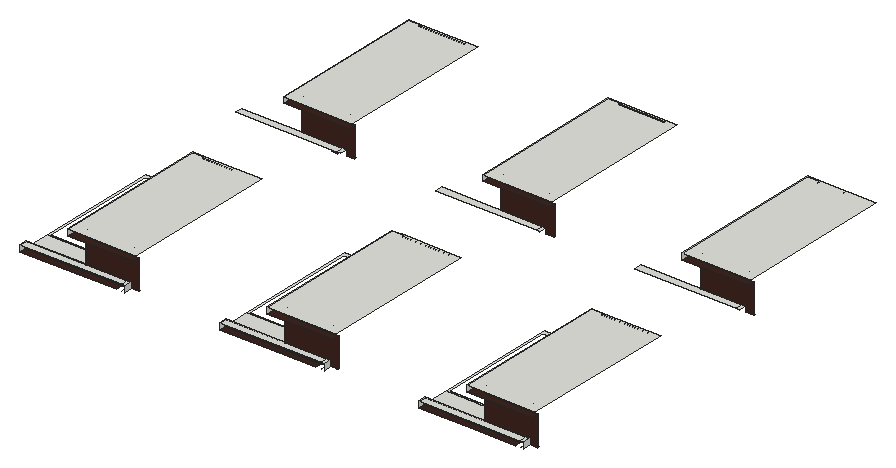
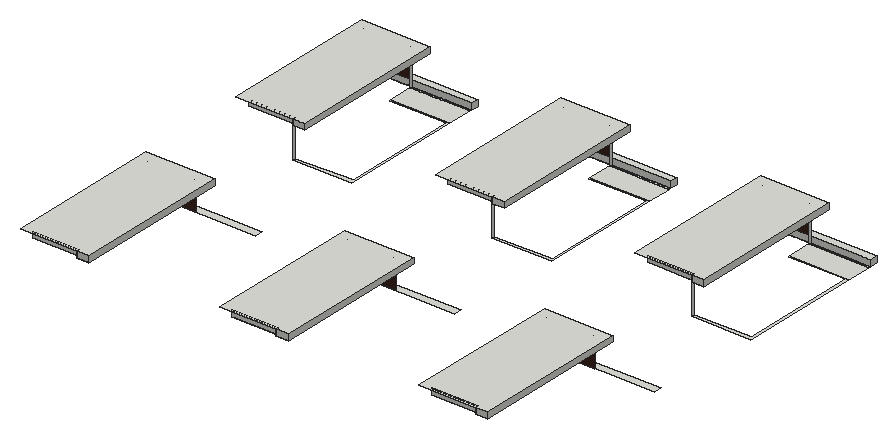
# SketchUp Ruby script. Lengths in inches.
U = 1.inch
M = Sketchup.active_model
def pt(a) = Geom::Point3d.new(a.map { |v| v * U })
def face(e, loops, mat)
  f = e.add_face(loops[0].map { |a| pt(a) })
  loops[1..].each { |l| e.add_face(l.map { |a| pt(a) }).erase! }
  f.material = f.back_material = mat if mat
  f
end
# faces: each face lists its corners as indices into pts; further lists are holes
def faces(e, pts, list, mat = nil) = list.each { |f| face(e, (f[0].is_a?(Array) ? f : [f]).map { |l| l.map { |i| pts[i] } }, mat) }
# xy, xz, yz: faces in a plane at the given z, y or x. An outline is a flat list of corners, or four numbers for a rectangle; further outlines are holes
def ring(l) = l.size == 4 ? [[l[0], l[1]], [l[2], l[1]], [l[2], l[3]], [l[0], l[3]]] : l.each_slice(2).to_a
def flat(e, list, mat, &to3) = list.each { |f| face(e, (f[0].is_a?(Array) ? f : [f]).map { |l| ring(l).map { |u, v| to3.(u, v) } }, mat) }
def xy(e, z, list, mat = nil) = flat(e, list, mat) { |x, y| [x, y, z] }
def xz(e, y, list, mat = nil) = flat(e, list, mat) { |x, z| [x, y, z] }
def yz(e, x, list, mat = nil) = flat(e, list, mat) { |y, z| [x, y, z] }
def lines(e, pts, list) = list.each { |a, b| e.add_line(pt(pts[a]), pt(pts[b])) }
# prism: a flat outline (further loops are holes) pulled along v
def prism(e, loops, v, mat = nil)
  f = face(e, loops, mat); d = Geom::Vector3d.new(v.map { |x| x * U })
  f.pushpull(f.normal.samedirection?(d) ? d.length : -d.length)
end
def box(e, o, s, mat = nil) = prism(e, [[o, [o[0] + s[0], o[1], o[2]], [o[0] + s[0], o[1] + s[1], o[2]], [o[0], o[1] + s[1], o[2]]]], [0, 0, s[2]], mat)
def at(x, y, z, deg = 0) = Geom::Transformation.translation(pt([x, y, z])) * Geom::Transformation.rotation(ORIGIN, Z_AXIS, deg.degrees)
def axes(o, x, y, z) = Geom::Transformation.new([*x, 0, *y, 0, *z, 0, *pt(o).to_a, 1])
def part(name) = M.definitions.add(name)
# library, detail: a bought-in or finely detailed component or shape, given as its bounding box
def library(name, o, s) = part(name).tap { |d| box(d.entities, o, s) }
def detail(e, o, s) = box(e.add_group.entities, o, s)
def put(e, d, t, mat = nil) = e.add_instance(d, t).tap { |i| i.material = mat if mat }
def group(e, t, mat = nil) = e.add_group.tap { |g| g.transformation = t; g.material = mat if mat }.entities
root = M.entities
M.materials.add("[0043_SaddleBrown]").color = [63, 38, 31]
xy(root,733.125,[[137.6,437.1,139.16,438.72],[139.16,437.1,143.93,438.72],[147.91,437.1,149.47,438.72],[149.47,437.1,154.24,438.72],[156.8,437.1,158.36,438.72],
  [158.36,437.1,163.14,438.72],[165.69,437.1,167.25,438.72],[167.25,437.1,172.03,438.72],[174.59,437.1,176.14,438.72],[176.14,437.1,180.92,438.72],
  [183.48,437.1,185.03,438.72],[185.03,437.1,189.81,438.72],[192.37,437.1,193.92,438.72],[193.92,437.1,198.7,438.72],[201.26,437.1,202.82,438.72],
  [202.82,437.1,207.59,438.72],[210.15,437.1,211.71,438.72],[211.71,437.1,216.48,438.72],[219.04,437.1,220.6,438.72],[220.6,437.1,225.375,438.72],
  [227.93,437.1,229.49,438.72],[229.49,437.1,234.27,438.72],[236.82,437.1,238.38,438.72],[238.38,437.1,243.16,438.72],[245.72,437.1,247.27,438.72],
  [247.27,437.1,252.05,438.72],[254.61,437.1,256.16,438.72],[256.16,437.1,260.94,438.72],[263.5,437.1,265.05,438.72],[265.05,437.1,269.83,438.72],
  [272.39,437.1,273.95,438.72],[273.95,437.1,278.72,438.72],[281.28,437.1,282.84,438.72],[282.84,437.1,287.61,438.72],[290.17,437.1,291.73,438.72],
  [291.73,437.1,296.51,438.72],[299.0625,437.1,300.62,438.72],[300.62,437.1,305.4,438.72],[307.95,437.1,309.51,438.72],[309.51,437.1,314.29,438.72],
  [316.85,437.1,318.4,438.72],[318.4,437.1,323.18,438.72],[325.74,437.1,327.29,438.72],[327.29,437.1,332.07,438.72],[334.63,437.1,336.19,438.72],
  [336.19,437.1,340.96,438.72],[343.52,437.1,345.08,438.72],[345.08,437.1,349.85,438.72],[352.41,437.1,353.97,438.72],[353.97,437.1,358.74,438.72],
  [361.3,437.1,367.0625,438.72],[369.3,437.1,375.0625,438.72],[377.3,437.1,383.0625,438.72],[385.3,437.1,391.0625,438.72],[393.3,437.1,399.0625,438.72],
  [401.3,437.1,407.0625,438.72],[409.3,437.1,415.0625,438.72],[417.3,437.1,423.0625,438.72],[425.3,437.1,431.0625,438.72],[433.3,437.1,439.0625,438.72],
  [441.3,437.1,447.0625,438.72],[449.3,437.1,455.0625,438.72],[457.3,437.1,463.0625,438.72],[465.3,437.1,471.0625,438.72],[473.3,437.1,479.0625,438.72],
  [481.3,437.1,487.0625,438.72],[862.04,437.1,863.59,438.72],[863.59,437.1,868.37,438.72],[872.35,437.1,873.91,438.72],[873.91,437.1,878.68,438.72],
  [881.24,437.1,882.8,438.72],[882.8,437.1,887.57,438.72],[890.13,437.1,891.6875,438.72],[891.6875,437.1,896.47,438.72],[899.02,437.1,900.58,438.72],
  [900.58,437.1,905.36,438.72],[907.91,437.1,909.47,438.72],[909.47,437.1,914.25,438.72],[916.81,437.1,918.36,438.72],[918.36,437.1,923.14,438.72],
  [925.7,437.1,927.25,438.72],[927.25,437.1,932.03,438.72],[934.59,437.1,936.14,438.72],[936.14,437.1,940.92,438.72],[943.48,437.1,945.04,438.72],
  [945.04,437.1,949.8125,438.72],[952.37,437.1,953.93,438.72],[953.93,437.1,958.7,438.72],[961.26,437.1,962.82,438.72],[962.82,437.1,967.6,438.72],
  [970.15,437.1,971.71,438.72],[971.71,437.1,976.49,438.72],[979.04,437.1,980.6,438.72],[980.6,437.1,985.38,438.72],[987.9375,437.1,989.49,438.72],
  [989.49,437.1,994.27,438.72],[996.83,437.1,998.38,438.72],[998.38,437.1,1003.16,438.72],[1005.72,437.1,1007.27,438.72],[1007.27,437.1,1012.05,438.72],
  [1014.61,437.1,1016.17,438.72],[1016.17,437.1,1020.94,438.72],[1023.5,437.1,1025.06,438.72],[1025.06,437.1,1029.83,438.72],[1032.39,437.1,1033.95,438.72],
  [1033.95,437.1,1038.73,438.72],[1041.28,437.1,1042.84,438.72],[1042.84,437.1,1047.62,438.72],[1050.17,437.1,1051.73,438.72],[1051.73,437.1,1056.51,438.72],
  [1059.07,437.1,1060.62,438.72],[1060.62,437.1,1065.4,438.72],[1067.96,437.1,1069.51,438.72],[1069.51,437.1,1074.29,438.72],[1076.85,437.1,1078.41,438.72],
  [1078.41,437.1,1083.18,438.72],[1085.74,437.1,1091.5,438.72],[1093.74,437.1,1099.5,438.72],[1101.74,437.1,1107.5,438.72],[1109.74,437.1,1115.5,438.72],
  [1117.74,437.1,1123.5,438.72],[1125.74,437.1,1131.5,438.72],[1133.74,437.1,1139.5,438.72],[1141.74,437.1,1147.5,438.72],[1149.74,437.1,1155.5,438.72],
  [1157.74,437.1,1163.5,438.72],[1165.74,437.1,1171.5,438.72],[1173.74,437.1,1179.5,438.72],[1181.74,437.1,1187.5,438.72],[1189.74,437.1,1195.5,438.72],
  [1197.74,437.1,1203.5,438.72],[1205.74,437.1,1211.5,438.72],[1586.47,437.1,1588.03,438.72],[1588.03,437.1,1592.81,438.72],[1596.79,437.1,1598.34,438.72],
  [1598.34,437.1,1603.12,438.72],[1605.68,437.1,1607.23,438.72],[1607.23,437.1,1612.01,438.72],[1614.57,437.1,1616.125,438.72],[1616.125,437.1,1620.9,438.72],
  [1623.46,437.1,1625.02,438.72],[1625.02,437.1,1629.79,438.72],[1632.35,437.1,1633.91,438.72],[1633.91,437.1,1638.69,438.72],[1641.24,437.1,1642.8,438.72],
  [1642.8,437.1,1647.58,438.72],[1650.13,437.1,1651.69,438.72],[1651.69,437.1,1656.47,438.72],[1659.03,437.1,1660.58,438.72],[1660.58,437.1,1665.36,438.72],
  [1667.92,437.1,1669.47,438.72],[1669.47,437.1,1674.25,438.72],[1676.81,437.1,1678.36,438.72],[1678.36,437.1,1683.14,438.72],[1685.7,437.1,1687.26,438.72],
  [1687.26,437.1,1692.03,438.72],[1694.59,437.1,1696.15,438.72],[1696.15,437.1,1700.92,438.72],[1703.48,437.1,1705.04,438.72],[1705.04,437.1,1709.82,438.72],
  [1712.375,437.1,1713.93,438.72],[1713.93,437.1,1718.71,438.72],[1721.26,437.1,1722.82,438.72],[1722.82,437.1,1727.6,438.72],[1730.16,437.1,1731.71,438.72],
  [1731.71,437.1,1736.49,438.72],[1739.05,437.1,1740.6,438.72],[1740.6,437.1,1745.38,438.72],[1747.9375,437.1,1749.5,438.72],[1749.5,437.1,1754.27,438.72],
  [1756.83,437.1,1758.39,438.72],[1758.39,437.1,1763.16,438.72],[1765.72,437.1,1767.28,438.72],[1767.28,437.1,1772.05,438.72],[1774.61,437.1,1776.17,438.72],
  [1776.17,437.1,1780.95,438.72],[1783.5,437.1,1785.06,438.72],[1785.06,437.1,1789.84,438.72],[1792.39,437.1,1793.95,438.72],[1793.95,437.1,1798.73,438.72],
  [1801.29,437.1,1802.84,438.72],[1802.84,437.1,1807.62,438.72],[1810.18,437.1,1815.9375,438.72],[1818.18,437.1,1823.9375,438.72],[1826.18,437.1,1831.9375,438.72],
  [1834.18,437.1,1839.9375,438.72],[1842.18,437.1,1847.9375,438.72],[1850.18,437.1,1855.9375,438.72],[1858.18,437.1,1863.9375,438.72],[1866.18,437.1,1871.9375,438.72],
  [1874.18,437.1,1879.9375,438.72],[1882.18,437.1,1887.9375,438.72],[1890.18,437.1,1895.9375,438.72],[1898.18,437.1,1903.9375,438.72],[1906.18,437.1,1911.9375,438.72],
  [1914.18,437.1,1919.9375,438.72],[1922.18,437.1,1927.9375,438.72],[1930.18,437.1,1935.9375,438.72],[137.5,438.72,353.97,447.84],[861.9375,438.72,1078.41,447.84],
  [1586.375,438.72,1802.84,447.84],[137.5,447.84,353.97,535.375],[861.9375,447.84,1078.41,535.375],[1586.375,447.84,1802.84,535.375],[137.5,535.375,353.97,535.375,353.97,540.48,144.84,540.48,144.84,965.96,353.97,971.23,353.97,980.35,137.5,980.35],
  [861.9375,535.375,1078.41,535.375,1078.41,540.48,869.28,540.48,869.28,965.96,1078.41,971.23,1078.41,980.35,861.9375,980.35],[1586.375,535.375,1802.84,535.375,1802.84,540.48,1593.72,540.48,1593.72,965.96,1802.84,971.23,1802.84,980.35,1586.375,980.35],[465.3,1417.45,471.0625,1419.07],[473.3,1417.45,479.0625,1419.07],[481.3,1417.45,487.0625,1419.07]])
xy(root,733.125,[[137.5,412.04,353.97,412.04,353.97,437.1,352.41,437.1,352.41,438.72,349.85,438.72,349.85,437.1,343.52,437.1,343.52,438.72,340.96,438.72,340.96,437.1,334.63,437.1,334.63,438.72,332.07,438.72,332.07,437.1,325.74,437.1,325.74,438.72,323.18,438.72,323.18,437.1,316.85,437.1,316.85,438.72,314.29,438.72,314.29,437.1,307.95,437.1,307.95,438.72,305.4,438.72,305.4,437.1,299.0625,437.1,299.0625,438.72,296.51,438.72,296.51,437.1,290.17,437.1,290.17,438.72,287.61,438.72,287.61,437.1,281.28,437.1,281.28,438.72,278.72,438.72,278.72,437.1,272.39,437.1,272.39,438.72,269.83,438.72,269.83,437.1,263.5,437.1,263.5,438.72,260.94,438.72,260.94,437.1,254.61,437.1,254.61,438.72,252.05,438.72,252.05,437.1,245.72,437.1,245.72,438.72,243.16,438.72,243.16,437.1,236.82,437.1,236.82,438.72,234.27,438.72,234.27,437.1,227.93,437.1,227.93,438.72,225.375,438.72,225.375,437.1,219.04,437.1,219.04,438.72,216.48,438.72,216.48,437.1,210.15,437.1,210.15,438.72,207.59,438.72,207.59,437.1,201.26,437.1,201.26,438.72,198.7,438.72,198.7,437.1,192.37,437.1,192.37,438.72,189.81,438.72,189.81,437.1,183.48,437.1,183.48,438.72,180.92,438.72,180.92,437.1,174.59,437.1,174.59,438.72,172.03,438.72,172.03,437.1,165.69,437.1,165.69,438.72,163.14,438.72,163.14,437.1,156.8,437.1,156.8,438.72,154.24,438.72,154.24,437.1,147.91,437.1,147.91,438.72,143.93,438.72,143.93,437.1,137.6,437.1,137.6,438.72,137.5,438.72],[353.97,412.04,353.97,437.1,358.74,437.1,358.74,438.72,361.3,438.72,361.3,437.1,367.0625,437.1,367.0625,438.72,369.3,438.72,369.3,437.1,375.0625,437.1,375.0625,438.72,377.3,438.72,377.3,437.1,383.0625,437.1,383.0625,438.72,385.3,438.72,385.3,437.1,391.0625,437.1,391.0625,438.72,393.3,438.72,393.3,437.1,399.0625,437.1,399.0625,438.72,401.3,438.72,401.3,437.1,407.0625,437.1,407.0625,438.72,409.3,438.72,409.3,437.1,415.0625,437.1,415.0625,438.72,417.3,438.72,417.3,437.1,423.0625,437.1,423.0625,438.72,425.3,438.72,425.3,437.1,431.0625,437.1,431.0625,438.72,433.3,438.72,433.3,437.1,439.0625,437.1,439.0625,438.72,441.3,438.72,441.3,437.1,447.0625,437.1,447.0625,438.72,449.3,438.72,449.3,437.1,455.0625,437.1,455.0625,438.72,457.3,438.72,457.3,437.1,463.0625,437.1,463.0625,438.72,465.3,438.72,465.3,437.1,471.0625,437.1,471.0625,438.72,473.3,438.72,473.3,437.1,479.0625,437.1,479.0625,438.72,481.3,438.72,481.3,437.1,487.0625,437.1,487.0625,412.04],[861.9375,412.04,1078.41,412.04,1078.41,437.1,1076.85,437.1,1076.85,438.72,1074.29,438.72,1074.29,437.1,1067.96,437.1,1067.96,438.72,1065.4,438.72,1065.4,437.1,1059.07,437.1,1059.07,438.72,1056.51,438.72,1056.51,437.1,1050.17,437.1,1050.17,438.72,1047.62,438.72,1047.62,437.1,1041.28,437.1,1041.28,438.72,1038.73,438.72,1038.73,437.1,1032.39,437.1,1032.39,438.72,1029.83,438.72,1029.83,437.1,1023.5,437.1,1023.5,438.72,1020.94,438.72,1020.94,437.1,1014.61,437.1,1014.61,438.72,1012.05,438.72,1012.05,437.1,1005.72,437.1,1005.72,438.72,1003.16,438.72,1003.16,437.1,996.83,437.1,996.83,438.72,994.27,438.72,994.27,437.1,987.9375,437.1,987.9375,438.72,985.38,438.72,985.38,437.1,979.04,437.1,979.04,438.72,976.49,438.72,976.49,437.1,970.15,437.1,970.15,438.72,967.6,438.72,967.6,437.1,961.26,437.1,961.26,438.72,958.7,438.72,958.7,437.1,952.37,437.1,952.37,438.72,949.8125,438.72,949.8125,437.1,943.48,437.1,943.48,438.72,940.92,438.72,940.92,437.1,934.59,437.1,934.59,438.72,932.03,438.72,932.03,437.1,925.7,437.1,925.7,438.72,923.14,438.72,923.14,437.1,916.81,437.1,916.81,438.72,914.25,438.72,914.25,437.1,907.91,437.1,907.91,438.72,905.36,438.72,905.36,437.1,899.02,437.1,899.02,438.72,896.47,438.72,896.47,437.1,890.13,437.1,890.13,438.72,887.57,438.72,887.57,437.1,881.24,437.1,881.24,438.72,878.68,438.72,878.68,437.1,872.35,437.1,872.35,438.72,868.37,438.72,868.37,437.1,862.04,437.1,862.04,438.72,861.9375,438.72],[1078.41,412.04,1078.41,437.1,1083.18,437.1,1083.18,438.72,1085.74,438.72,1085.74,437.1,1091.5,437.1,1091.5,438.72,1093.74,438.72,1093.74,437.1,1099.5,437.1,1099.5,438.72,1101.74,438.72,1101.74,437.1,1107.5,437.1,1107.5,438.72,1109.74,438.72,1109.74,437.1,1115.5,437.1,1115.5,438.72,1117.74,438.72,1117.74,437.1,1123.5,437.1,1123.5,438.72,1125.74,438.72,1125.74,437.1,1131.5,437.1,1131.5,438.72,1133.74,438.72,1133.74,437.1,1139.5,437.1,1139.5,438.72,1141.74,438.72,1141.74,437.1,1147.5,437.1,1147.5,438.72,1149.74,438.72,1149.74,437.1,1155.5,437.1,1155.5,438.72,1157.74,438.72,1157.74,437.1,1163.5,437.1,1163.5,438.72,1165.74,438.72,1165.74,437.1,1171.5,437.1,1171.5,438.72,1173.74,438.72,1173.74,437.1,1179.5,437.1,1179.5,438.72,1181.74,438.72,1181.74,437.1,1187.5,437.1,1187.5,438.72,1189.74,438.72,1189.74,437.1,1195.5,437.1,1195.5,438.72,1197.74,438.72,1197.74,437.1,1203.5,437.1,1203.5,438.72,1205.74,438.72,1205.74,437.1,1211.5,437.1,1211.5,412.04],[1586.375,412.04,1802.84,412.04,1802.84,437.1,1801.29,437.1,1801.29,438.72,1798.73,438.72,1798.73,437.1,1792.39,437.1,1792.39,438.72,1789.84,438.72,1789.84,437.1,1783.5,437.1,1783.5,438.72,1780.95,438.72,1780.95,437.1,1774.61,437.1,1774.61,438.72,1772.05,438.72,1772.05,437.1,1765.72,437.1,1765.72,438.72,1763.16,438.72,1763.16,437.1,1756.83,437.1,1756.83,438.72,1754.27,438.72,1754.27,437.1,1747.9375,437.1,1747.9375,438.72,1745.38,438.72,1745.38,437.1,1739.05,437.1,1739.05,438.72,1736.49,438.72,1736.49,437.1,1730.16,437.1,1730.16,438.72,1727.6,438.72,1727.6,437.1,1721.26,437.1,1721.26,438.72,1718.71,438.72,1718.71,437.1,1712.375,437.1,1712.375,438.72,1709.82,438.72,1709.82,437.1,1703.48,437.1,1703.48,438.72,1700.92,438.72,1700.92,437.1,1694.59,437.1,1694.59,438.72,1692.03,438.72,1692.03,437.1,1685.7,437.1,1685.7,438.72,1683.14,438.72,1683.14,437.1,1676.81,437.1,1676.81,438.72,1674.25,438.72,1674.25,437.1,1667.92,437.1,1667.92,438.72,1665.36,438.72,1665.36,437.1,1659.03,437.1,1659.03,438.72,1656.47,438.72,1656.47,437.1,1650.13,437.1,1650.13,438.72,1647.58,438.72,1647.58,437.1,1641.24,437.1,1641.24,438.72,1638.69,438.72,1638.69,437.1,1632.35,437.1,1632.35,438.72,1629.79,438.72,1629.79,437.1,1623.46,437.1,1623.46,438.72,1620.9,438.72,1620.9,437.1,1614.57,437.1,1614.57,438.72,1612.01,438.72,1612.01,437.1,1605.68,437.1,1605.68,438.72,1603.12,438.72,1603.12,437.1,1596.79,437.1,1596.79,438.72,1592.81,438.72,1592.81,437.1,1586.47,437.1,1586.47,438.72,1586.375,438.72],
  [1802.84,412.04,1802.84,437.1,1807.62,437.1,1807.62,438.72,1810.18,438.72,1810.18,437.1,1815.9375,437.1,1815.9375,438.72,1818.18,438.72,1818.18,437.1,1823.9375,437.1,1823.9375,438.72,1826.18,438.72,1826.18,437.1,1831.9375,437.1,1831.9375,438.72,1834.18,438.72,1834.18,437.1,1839.9375,437.1,1839.9375,438.72,1842.18,438.72,1842.18,437.1,1847.9375,437.1,1847.9375,438.72,1850.18,438.72,1850.18,437.1,1855.9375,437.1,1855.9375,438.72,1858.18,438.72,1858.18,437.1,1863.9375,437.1,1863.9375,438.72,1866.18,438.72,1866.18,437.1,1871.9375,437.1,1871.9375,438.72,1874.18,438.72,1874.18,437.1,1879.9375,437.1,1879.9375,438.72,1882.18,438.72,1882.18,437.1,1887.9375,437.1,1887.9375,438.72,1890.18,438.72,1890.18,437.1,1895.9375,437.1,1895.9375,438.72,1898.18,438.72,1898.18,437.1,1903.9375,437.1,1903.9375,438.72,1906.18,438.72,1906.18,437.1,1911.9375,437.1,1911.9375,438.72,1914.18,438.72,1914.18,437.1,1919.9375,437.1,1919.9375,438.72,1922.18,438.72,1922.18,437.1,1927.9375,437.1,1927.9375,438.72,1930.18,438.72,1930.18,437.1,1935.9375,437.1,1935.9375,412.04]],"[0043_SaddleBrown]")
xy(root,736,[[517.3125,438.72,517.3125,442.66,547.05,442.66,547.05,438.73],[1241.75,438.72,1241.75,442.66,1271.49,442.66,1271.49,438.73],[1966.1875,438.72,1966.1875,442.66,1995.93,442.66,1995.93,438.73],[517.3125,1419.07,517.3125,1423.01,547.05,1423.01,547.05,1419.08],[1241.75,1419.07,1241.75,1423.01,1271.49,1423.01,1271.49,1419.08],
  [1966.1875,1419.07,1966.1875,1423.01,1995.93,1423.01,1995.93,1419.08]])
xy(root,755.5,[[137.5,412.04,504.5,438.72],[504.5,412.04,517.3125,438.72],[861.9375,412.04,1228.9375,438.72],[1228.9375,412.04,1241.75,438.72],[1586.375,412.04,1953.375,438.72],
  [1953.375,412.04,1966.1875,438.72],[137.5,1392.39,504.5,1419.07],[504.5,1392.39,517.3125,1419.07],[861.9375,1392.39,1228.9375,1419.07],[1228.9375,1392.39,1241.75,1419.07],
  [1586.375,1392.39,1953.375,1419.07],[1953.375,1392.39,1966.1875,1419.07]])
xy(root,845.41,[[353.97,447.84,521.63,971.23],[1078.41,447.84,1246.07,971.23],[1802.84,447.84,1970.51,971.23],[353.97,1428.19,521.63,1951.58],[1078.41,1428.19,1246.07,1951.58],
  [1802.84,1428.19,1970.51,1951.58]])
xy(root,845.41,[[308.59,412.04,308.59,980.35,353.97,980.35,353.97,438.72,547.05,438.72,547.05,412.04],[1033.03,412.04,1033.03,980.35,1078.41,980.35,1078.41,438.72,1271.49,438.72,1271.49,412.04],[1757.47,412.04,1757.47,980.35,1802.84,980.35,1802.84,438.72,1995.93,438.72,1995.93,412.04],[308.59,1392.39,308.59,1960.7,353.97,1960.7,353.97,1419.07,547.05,1419.07,547.05,1392.39],[1033.03,1392.39,1033.03,1960.7,1078.41,1960.7,1078.41,1419.07,1271.49,1419.07,1271.49,1392.39],
  [1757.47,1392.39,1757.47,1960.7,1802.84,1960.7,1802.84,1419.07,1995.93,1419.07,1995.93,1392.39]],"[0043_SaddleBrown]")
xy(root,866.5625,[[308.59,412.04,558.625,412.04,558.625,980.35,353.97,980.35,353.97,971.23,353.97,980.35,308.59,980.35],[1033.03,412.04,1283.0625,412.04,1283.0625,980.35,1078.41,980.35,1078.41,971.23,1078.41,980.35,1033.03,980.35],[1757.47,412.04,2007.5,412.04,2007.5,980.35,1802.84,980.35,1802.84,971.23,1802.84,980.35,1757.47,980.35],[308.59,1392.39,558.625,1392.39,558.625,1960.7,353.97,1960.7,353.97,1951.58,353.97,1960.7,308.59,1960.7],[1033.03,1392.39,1283.0625,1392.39,1283.0625,1960.7,1078.41,1960.7,1078.41,1951.58,1078.41,1960.7,1033.03,1960.7],
  [1757.47,1392.39,2007.5,1392.39,2007.5,1960.7,1802.84,1960.7,1802.84,1951.58,1802.84,1960.7,1757.47,1960.7]])
xz(root,438.72,[[137.5,733.125,353.97,755.5],[353.97,733.125,487.0625,755.5],[487.0625,733.125,504.5,755.5],[504.5,733.125,517.3125,755.5],[861.9375,733.125,1078.41,755.5],
  [1078.41,733.125,1211.5,755.5],[1211.5,733.125,1228.9375,755.5],[1228.9375,733.125,1241.75,755.5],[1586.375,733.125,1802.84,755.5],[1802.84,733.125,1935.9375,755.5],
  [1935.9375,733.125,1953.375,755.5],[1953.375,733.125,1966.1875,755.5]])
xz(root,971.23,[[353.97,845.41,521.63,866.5625],[1078.41,845.41,1246.07,866.5625],[1802.84,845.41,1970.51,866.5625]])
xz(root,980.35,[[308.59,845.41,353.97,866.5625],[1033.03,845.41,1078.41,866.5625],[1757.47,845.41,1802.84,866.5625]])
xz(root,1951.58,[[353.97,845.41,521.63,866.5625],[1078.41,845.41,1246.07,866.5625],[1802.84,845.41,1970.51,866.5625]])
xz(root,1960.7,[[308.59,845.41,353.97,866.5625],[1033.03,845.41,1078.41,866.5625],[1757.47,845.41,1802.84,866.5625]])
yz(root,137.5,[[412.04,733.125,438.72,755.5]])
yz(root,308.59,[[412.04,845.41,980.35,866.5625],[1392.39,845.41,1960.7,866.5625]])
yz(root,353.97,[[438.72,733.125,447.84,845.41],[971.23,733.125,980.35,845.41],[971.23,845.41,980.35,866.5625],[1951.58,845.41,1960.7,866.5625]])
yz(root,517.3125,[[412.04,733.125,438.72,755.5]])
yz(root,861.9375,[[412.04,733.125,438.72,755.5]])
yz(root,1033.03,[[412.04,845.41,980.35,866.5625],[1392.39,845.41,1960.7,866.5625]])
yz(root,1078.41,[[438.72,733.125,447.84,845.41],[971.23,733.125,980.35,845.41],[971.23,845.41,980.35,866.5625],[1951.58,845.41,1960.7,866.5625]])
yz(root,1241.75,[[412.04,733.125,438.72,755.5]])
yz(root,1586.375,[[412.04,733.125,438.72,755.5]])
yz(root,1757.47,[[412.04,845.41,980.35,866.5625],[1392.39,845.41,1960.7,866.5625]])
yz(root,1802.84,[[438.72,733.125,447.84,845.41],[971.23,733.125,980.35,845.41],[971.23,845.41,980.35,866.5625],[1951.58,845.41,1960.7,866.5625]])
yz(root,1966.1875,[[412.04,733.125,438.72,755.5]])
p = [[517.3125,438.72,755.5],[517.3125,438.72,736],[547.05,438.73,736],[547.05,438.72,845.41],[353.97,438.72,845.41],[353.97,438.72,755.5],
  [487.0625,438.72,755.5],[504.5,438.72,755.5],[1241.75,438.72,755.5],[1241.75,438.72,736],[1271.49,438.73,736],[1271.49,438.72,845.41],
  [1078.41,438.72,845.41],[1078.41,438.72,755.5],[1211.5,438.72,755.5],[1228.9375,438.72,755.5],[1966.1875,438.72,755.5],[1966.1875,438.72,736],
  [1995.93,438.73,736],[1995.93,438.72,845.41],[1802.84,438.72,845.41],[1802.84,438.72,755.5],[1935.9375,438.72,755.5],[1953.375,438.72,755.5],
  [517.3125,1419.07,755.5],[517.3125,1419.07,736],[547.05,1419.08,736],[547.05,1419.07,845.41],[353.97,1419.07,845.41],[353.97,1419.07,755.5],
  [487.0625,1419.07,755.5],[504.5,1419.07,755.5],[1241.75,1419.07,755.5],[1241.75,1419.07,736],[1271.49,1419.08,736],[1271.49,1419.07,845.41],
  [1078.41,1419.07,845.41],[1078.41,1419.07,755.5],[1211.5,1419.07,755.5],[1228.9375,1419.07,755.5],[1966.1875,1419.07,755.5],[1966.1875,1419.07,736],
  [1995.93,1419.08,736],[1995.93,1419.07,845.41],[1802.84,1419.07,845.41],[1802.84,1419.07,755.5],[1935.9375,1419.07,755.5],[1953.375,1419.07,755.5],
  [1228.9375,438.72,733.125],[1228.9375,412.04,733.125],[1078.41,447.84,845.41],[1078.41,447.84,866.5625],[1246.07,447.84,845.41],[1246.07,447.84,866.5625],
  [1953.375,438.72,733.125],[1953.375,412.04,733.125],[1802.84,447.84,845.41],[1802.84,447.84,866.5625],[1970.51,447.84,845.41],[1970.51,447.84,866.5625],
  [353.97,447.84,845.41],[353.97,447.84,866.5625],[521.63,447.84,845.41],[521.63,447.84,866.5625],[504.5,438.72,733.125],[504.5,412.04,733.125],
  [1078.41,1428.19,845.41],[1078.41,1428.19,866.5625],[1246.07,1428.19,845.41],[1246.07,1428.19,866.5625],[1802.84,1428.19,845.41],[1802.84,1428.19,866.5625],
  [1970.51,1428.19,845.41],[1970.51,1428.19,866.5625],[353.97,1428.19,845.41],[353.97,1428.19,866.5625],[521.63,1428.19,845.41],[521.63,1428.19,866.5625]]
faces(root,p,[[0,1,2,3,4,5,6,7],[8,9,10,11,12,13,14,15],[16,17,18,19,20,21,22,23],[24,25,26,27,28,29,30,31],[32,33,34,35,36,37,38,39],[40,41,42,43,44,45,46,47]],"[0043_SaddleBrown]")
lines(root,p,[[48,49],[50,51],[52,53],[54,55],[56,57],[58,59],[60,61],[62,63],[64,65],[66,67],[68,69],[70,71],
  [72,73],[74,75],[76,77]])
